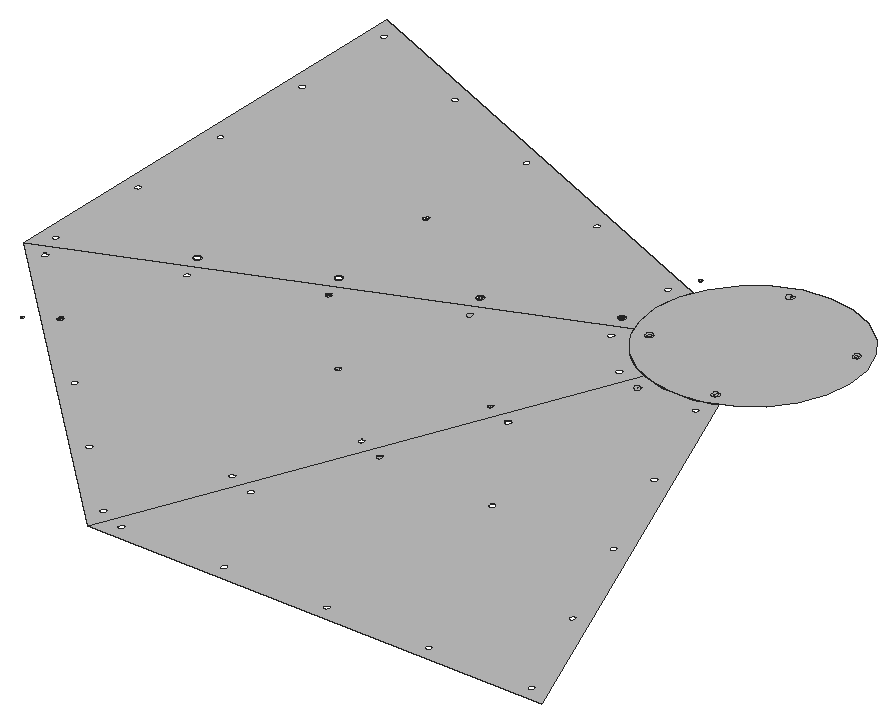
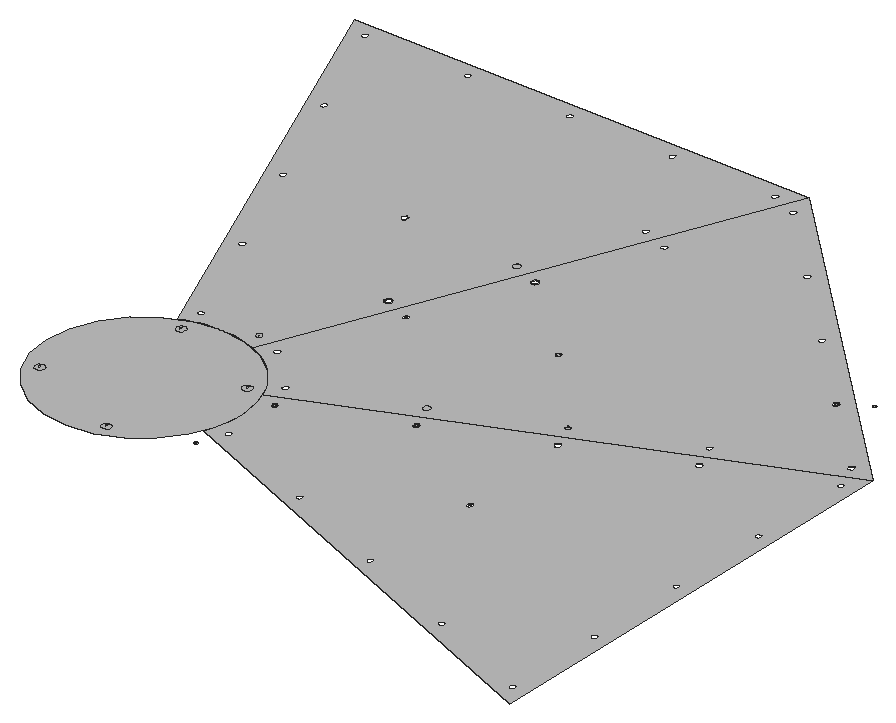
# SketchUp Ruby script. Lengths in inches.
U = 1.inch
M = Sketchup.active_model
def pt(a) = Geom::Point3d.new(a.map { |v| v * U })
def face(e, loops, mat)
  f = e.add_face(loops[0].map { |a| pt(a) })
  loops[1..].each { |l| e.add_face(l.map { |a| pt(a) }).erase! }
  f.material = f.back_material = mat if mat
  f
end
# faces: each face lists its corners as indices into pts; further lists are holes
def faces(e, pts, list, mat = nil) = list.each { |f| face(e, (f[0].is_a?(Array) ? f : [f]).map { |l| l.map { |i| pts[i] } }, mat) }
# xy, xz, yz: faces in a plane at the given z, y or x. An outline is a flat list of corners, or four numbers for a rectangle; further outlines are holes
def ring(l) = l.size == 4 ? [[l[0], l[1]], [l[2], l[1]], [l[2], l[3]], [l[0], l[3]]] : l.each_slice(2).to_a
def flat(e, list, mat, &to3) = list.each { |f| face(e, (f[0].is_a?(Array) ? f : [f]).map { |l| ring(l).map { |u, v| to3.(u, v) } }, mat) }
def xy(e, z, list, mat = nil) = flat(e, list, mat) { |x, y| [x, y, z] }
def xz(e, y, list, mat = nil) = flat(e, list, mat) { |x, z| [x, y, z] }
def yz(e, x, list, mat = nil) = flat(e, list, mat) { |y, z| [x, y, z] }
def lines(e, pts, list) = list.each { |a, b| e.add_line(pt(pts[a]), pt(pts[b])) }
# prism: a flat outline (further loops are holes) pulled along v
def prism(e, loops, v, mat = nil)
  f = face(e, loops, mat); d = Geom::Vector3d.new(v.map { |x| x * U })
  f.pushpull(f.normal.samedirection?(d) ? d.length : -d.length)
end
def box(e, o, s, mat = nil) = prism(e, [[o, [o[0] + s[0], o[1], o[2]], [o[0] + s[0], o[1] + s[1], o[2]], [o[0], o[1] + s[1], o[2]]]], [0, 0, s[2]], mat)
def at(x, y, z, deg = 0) = Geom::Transformation.translation(pt([x, y, z])) * Geom::Transformation.rotation(ORIGIN, Z_AXIS, deg.degrees)
def axes(o, x, y, z) = Geom::Transformation.new([*x, 0, *y, 0, *z, 0, *pt(o).to_a, 1])
def part(name) = M.definitions.add(name)
# library, detail: a bought-in or finely detailed component or shape, given as its bounding box
def library(name, o, s) = part(name).tap { |d| box(d.entities, o, s) }
def detail(e, o, s) = box(e.add_group.entities, o, s)
def put(e, d, t, mat = nil) = e.add_instance(d, t).tap { |i| i.material = mat if mat }
def group(e, t, mat = nil) = e.add_group.tap { |g| g.transformation = t; g.material = mat if mat }.entities
root = M.entities
M.materials.add("[Metal_Steel_Textured_White]").color = [191, 191, 191]
xy(root,3.625,[[[143.617,148.407,134.847,157.176,147.359,162.359,147.431,162.2,147.513,162.047,147.605,161.899,147.706,161.757,147.817,161.623,147.936,161.495,148.063,161.376,148.198,161.266,148.339,161.165,148.487,161.073,148.641,160.99,148.799,160.919],[147.085,157.734,147.108,157.737,147.129,157.746,147.148,157.76,147.162,157.778,147.171,157.8,147.174,157.823,147.171,157.846,147.162,157.867,147.148,157.886,147.129,157.9,147.108,157.909,147.085,157.912,147.062,157.909,147.041,157.9,147.022,157.886,147.008,157.867,146.999,157.846,146.996,157.823,146.999,157.8,147.008,157.778,147.022,157.76,147.041,157.746,147.062,157.737],[141.36,159.353,141.383,159.356,141.404,159.365,141.422,159.379,141.437,159.397,141.445,159.419,141.448,159.442,141.445,159.465,141.437,159.486,141.422,159.505,141.404,159.519,141.383,159.528,141.36,159.531,141.337,159.528,141.315,159.519,141.297,159.505,141.283,159.486,141.274,159.465,141.271,159.442,141.274,159.419,141.283,159.397,141.297,159.379,141.315,159.365,141.337,159.356],[141.495,151.004,141.518,151.007,141.54,151.016,141.558,151.03,141.572,151.048,141.581,151.07,141.584,151.093,141.581,151.116,141.572,151.137,141.558,151.156,141.54,151.17,141.518,151.179,141.495,151.182,141.472,151.179,141.451,151.17,141.433,151.156,141.418,151.137,141.41,151.116,141.407,151.093,141.41,151.07,141.418,151.048,141.433,151.03,141.451,151.016,141.472,151.007],[135.552,156.947,135.575,156.95,135.596,156.959,135.615,156.973,135.629,156.992,135.638,157.013,135.641,157.036,135.638,157.059,135.629,157.081,135.615,157.099,135.596,157.113,135.575,157.122,135.552,157.125,135.529,157.122,135.508,157.113,135.489,157.099,135.475,157.081,135.466,157.059,135.463,157.036,135.466,157.013,135.475,156.992,135.489,156.973,135.508,156.959,135.529,156.95],[144.263,160.556,144.286,160.559,144.308,160.568,144.326,160.582,144.34,160.6,144.349,160.622,144.352,160.645,144.349,160.668,144.34,160.689,144.326,160.707,144.308,160.722,144.286,160.73,144.263,160.733,144.24,160.73,144.219,160.722,144.2,160.707,144.186,160.689,144.177,160.668,144.174,160.645,144.177,160.622,144.186,160.6,144.2,160.582,144.219,160.568,144.24,160.559],[143.477,149.023,143.5,149.026,143.521,149.035,143.539,149.049,143.554,149.067,143.5625,149.088,143.566,149.112,143.5625,149.135,143.554,149.156,143.539,149.174,143.521,149.188,143.5,149.197,143.477,149.2,143.454,149.197,143.432,149.188,143.414,149.174,143.4,149.156,143.391,149.135,143.388,149.112,143.391,149.088,143.4,149.067,143.414,149.049,143.432,149.035,143.454,149.026],[138.456,158.15,138.479,158.153,138.5,158.162,138.519,158.176,138.533,158.195,138.542,158.216,138.545,158.239,138.542,158.262,138.533,158.283,138.519,158.302,138.5,158.316,138.479,158.325,138.456,158.328,138.433,158.325,138.411,158.316,138.393,158.302,138.379,158.283,138.37,158.262,138.367,158.239,138.37,158.216,138.379,158.195,138.393,158.176,138.411,158.162,138.433,158.153],[145.882,154.83,145.905,154.833,145.927,154.842,145.945,154.856,145.959,154.875,145.968,154.896,145.971,154.919,145.968,154.942,145.959,154.964,145.945,154.982,145.927,154.996,145.905,155.005,145.882,155.008,145.859,155.005,145.838,154.996,145.819,154.982,145.805,154.964,145.796,154.942,145.793,154.919,145.796,154.896,145.805,154.875,145.819,154.856,145.838,154.842,145.859,154.833],[148.288,160.638,148.311,160.641,148.332,160.65,148.351,160.664,148.365,160.682,148.374,160.704,148.377,160.727,148.374,160.75,148.365,160.771,148.351,160.79,148.332,160.804,148.311,160.8125,148.288,160.816,148.265,160.8125,148.243,160.804,148.225,160.79,148.211,160.771,148.202,160.75,148.199,160.727,148.202,160.704,148.211,160.682,148.225,160.664,148.243,160.65,148.265,160.641],[147.167,161.758,147.19,161.761,147.212,161.77,147.23,161.784,147.244,161.803,147.253,161.824,147.256,161.847,147.253,161.87,147.244,161.892,147.23,161.91,147.212,161.924,147.19,161.933,147.167,161.936,147.144,161.933,147.123,161.924,147.104,161.91,147.09,161.892,147.081,161.87,147.078,161.847,147.081,161.824,147.09,161.803,147.104,161.784,147.123,161.77,147.144,161.761],[144.679,151.926,144.702,151.929,144.724,151.938,144.742,151.952,144.756,151.971,144.765,151.992,144.768,152.015,144.765,152.038,144.756,152.06,144.742,152.078,144.724,152.092,144.702,152.101,144.679,152.104,144.656,152.101,144.635,152.092,144.617,152.078,144.602,152.06,144.594,152.038,144.591,152.015,144.594,151.992,144.602,151.971,144.617,151.952,144.635,151.938,144.656,151.929],[139.514,152.985,139.537,152.988,139.559,152.997,139.577,153.011,139.591,153.029,139.6,153.051,139.603,153.074,139.6,153.097,139.591,153.118,139.577,153.137,139.559,153.151,139.537,153.16,139.514,153.163,139.491,153.16,139.47,153.151,139.451,153.137,139.4375,153.118,139.428,153.097,139.425,153.074,139.428,153.051,139.4375,153.029,139.451,153.011,139.47,152.997,139.491,152.988],[137.533,154.966,137.556,154.969,137.578,154.978,137.596,154.992,137.61,155.011,137.619,155.032,137.622,155.055,137.619,155.078,137.61,155.099,137.596,155.118,137.578,155.132,137.556,155.141,137.533,155.144,137.51,155.141,137.489,155.132,137.47,155.118,137.456,155.099,137.447,155.078,137.444,155.055,137.447,155.032,137.456,155.011,137.47,154.992,137.489,154.978,137.51,154.969],[143.513,156.984,143.536,156.987,143.558,156.996,143.576,157.01,143.59,157.029,143.599,157.05,143.602,157.073,143.599,157.096,143.59,157.117,143.576,157.136,143.558,157.15,143.536,157.159,143.513,157.162,143.49,157.159,143.469,157.15,143.451,157.136,143.436,157.117,143.428,157.096,143.425,157.073,143.428,157.05,143.436,157.029,143.451,157.01,143.469,156.996,143.49,156.987]],[[143.617,148.407,148.799,160.919,148.962,160.857,149.129,160.807,149.299,160.767,149.471,160.739,149.644,160.722,149.818,160.716,149.992,160.722,150.165,160.739,150.337,160.767,150.507,160.807,150.673,160.857,150.836,160.919,156.019,148.407],[154.219,151.621,154.242,151.624,154.263,151.633,154.282,151.647,154.296,151.665,154.305,151.687,154.308,151.71,154.305,151.733,154.296,151.754,154.282,151.773,154.263,151.787,154.242,151.796,154.219,151.799,154.196,151.796,154.174,151.787,154.156,151.773,154.142,151.754,154.133,151.733,154.13,151.71,154.133,151.687,154.142,151.665,154.156,151.647,154.174,151.633,154.196,151.624],[145.417,151.621,145.44,151.624,145.462,151.633,145.48,151.647,145.494,151.665,145.503,151.687,145.506,151.71,145.503,151.733,145.494,151.754,145.48,151.773,145.462,151.787,145.44,151.796,145.417,151.799,145.394,151.796,145.373,151.787,145.354,151.773,145.34,151.754,145.331,151.733,145.328,151.71,145.331,151.687,145.34,151.665,145.354,151.647,145.373,151.633,145.394,151.624],[149.025,160.332,149.048,160.335,149.07,160.344,149.088,160.358,149.102,160.377,149.111,160.398,149.114,160.421,149.111,160.444,149.102,160.466,149.088,160.484,149.07,160.498,149.048,160.507,149.025,160.51,149.002,160.507,148.981,160.498,148.963,160.484,148.948,160.466,148.94,160.444,148.937,160.421,148.94,160.398,148.948,160.377,148.963,160.358,148.981,160.344,149.002,160.335],[155.421,148.717,155.444,148.72,155.466,148.729,155.484,148.743,155.498,148.762,155.507,148.783,155.51,148.806,155.507,148.829,155.498,148.85,155.484,148.869,155.466,148.883,155.444,148.892,155.421,148.895,155.398,148.892,155.377,148.883,155.359,148.869,155.345,148.85,155.336,148.829,155.333,148.806,155.336,148.783,155.345,148.762,155.359,148.743,155.377,148.729,155.398,148.72],[147.823,157.428,147.846,157.431,147.867,157.44,147.886,157.454,147.9,157.473,147.909,157.494,147.912,157.517,147.909,157.54,147.9,157.562,147.886,157.58,147.867,157.594,147.846,157.603,147.823,157.606,147.8,157.603,147.778,157.594,147.76,157.58,147.746,157.562,147.737,157.54,147.734,157.517,147.737,157.494,147.746,157.473,147.76,157.454,147.778,157.44,147.8,157.431],[144.214,148.717,144.237,148.72,144.259,148.729,144.277,148.743,144.291,148.762,144.3,148.783,144.303,148.806,144.3,148.829,144.291,148.85,144.277,148.869,144.259,148.883,144.237,148.892,144.214,148.895,144.191,148.892,144.17,148.883,144.151,148.869,144.137,148.85,144.128,148.829,144.125,148.806,144.128,148.783,144.137,148.762,144.151,148.743,144.17,148.729,144.191,148.72],[150.61,160.332,150.633,160.335,150.655,160.344,150.673,160.358,150.6875,160.377,150.696,160.398,150.699,160.421,150.696,160.444,150.6875,160.466,150.673,160.484,150.655,160.498,150.633,160.507,150.61,160.51,150.587,160.507,150.566,160.498,150.547,160.484,150.533,160.466,150.524,160.444,150.521,160.421,150.524,160.398,150.533,160.377,150.547,160.358,150.566,160.344,150.587,160.335],[149.818,154.373,149.841,154.376,149.862,154.385,149.881,154.399,149.895,154.417,149.904,154.439,149.907,154.462,149.904,154.485,149.895,154.506,149.881,154.524,149.862,154.539,149.841,154.547,149.818,154.55,149.795,154.547,149.773,154.539,149.755,154.524,149.741,154.506,149.732,154.485,149.729,154.462,149.732,154.439,149.741,154.417,149.755,154.399,149.773,154.385,149.795,154.376],[153.016,154.525,153.039,154.528,153.06,154.537,153.079,154.551,153.093,154.569,153.102,154.591,153.105,154.614,153.102,154.637,153.093,154.658,153.079,154.676,153.06,154.691,153.039,154.699,153.016,154.702,152.993,154.699,152.971,154.691,152.953,154.676,152.939,154.658,152.93,154.637,152.927,154.614,152.93,154.591,152.939,154.569,152.953,154.551,152.971,154.537,152.993,154.528],[147.016,148.717,147.039,148.72,147.061,148.729,147.079,148.743,147.093,148.762,147.102,148.783,147.105,148.806,147.102,148.829,147.093,148.85,147.079,148.869,147.061,148.883,147.039,148.892,147.016,148.895,146.993,148.892,146.972,148.883,146.953,148.869,146.939,148.85,146.93,148.829,146.927,148.806,146.93,148.783,146.939,148.762,146.953,148.743,146.972,148.729,146.993,148.72],[149.818,148.717,149.841,148.72,149.862,148.729,149.881,148.743,149.895,148.762,149.904,148.783,149.907,148.806,149.904,148.829,149.895,148.85,149.881,148.869,149.862,148.883,149.841,148.892,149.818,148.895,149.795,148.892,149.773,148.883,149.755,148.869,149.741,148.85,149.732,148.829,149.729,148.806,149.732,148.783,149.741,148.762,149.755,148.743,149.773,148.729,149.795,148.72],[152.62,148.717,152.643,148.72,152.664,148.729,152.683,148.743,152.697,148.762,152.706,148.783,152.709,148.806,152.706,148.829,152.697,148.85,152.683,148.869,152.664,148.883,152.643,148.892,152.62,148.895,152.597,148.892,152.575,148.883,152.557,148.869,152.543,148.85,152.534,148.829,152.531,148.806,152.534,148.783,152.543,148.762,152.557,148.743,152.575,148.729,152.597,148.72],[146.62,154.525,146.643,154.528,146.664,154.537,146.683,154.551,146.697,154.569,146.706,154.591,146.709,154.614,146.706,154.637,146.697,154.658,146.683,154.676,146.664,154.691,146.643,154.699,146.62,154.702,146.597,154.699,146.575,154.691,146.557,154.676,146.543,154.658,146.534,154.637,146.531,154.614,146.534,154.591,146.543,154.569,146.557,154.551,146.575,154.537,146.597,154.528],[151.813,157.428,151.836,157.431,151.858,157.44,151.876,157.454,151.89,157.473,151.899,157.494,151.902,157.517,151.899,157.54,151.89,157.562,151.876,157.58,151.858,157.594,151.836,157.603,151.813,157.606,151.79,157.603,151.769,157.594,151.75,157.58,151.736,157.562,151.727,157.54,151.724,157.517,151.727,157.494,151.736,157.473,151.75,157.454,151.769,157.44,151.79,157.431]],[149.818,154.373,149.795,154.376,149.773,154.385,149.755,154.399,149.741,154.417,149.732,154.439,149.729,154.462,149.732,154.485,149.741,154.506,149.755,154.524,149.773,154.539,149.795,154.547,149.818,154.55,149.818,154.549,149.795,154.546,149.774,154.538,149.756,154.524,149.742,154.506,149.733,154.484,149.73,154.462,149.733,154.439,149.742,154.418,149.756,154.399,149.774,154.385,149.795,154.377,149.818,154.374],[[146.62,154.525,146.597,154.528,146.575,154.537,146.557,154.551,146.543,154.569,146.534,154.591,146.531,154.614,146.534,154.637,146.543,154.658,146.557,154.676,146.575,154.691,146.597,154.699,146.62,154.702,146.643,154.699,146.664,154.691,146.683,154.676,146.697,154.658,146.706,154.637,146.709,154.614,146.706,154.591,146.697,154.569,146.683,154.551,146.664,154.537,146.643,154.528],[146.62,154.526,146.643,154.529,146.664,154.537,146.682,154.551,146.696,154.57,146.705,154.591,146.708,154.614,146.705,154.636,146.696,154.657,146.682,154.676,146.664,154.69,146.643,154.698,146.62,154.701,146.597,154.698,146.576,154.69,146.558,154.676,146.544,154.657,146.535,154.636,146.532,154.614,146.535,154.591,146.544,154.57,146.558,154.551,146.576,154.537,146.597,154.529]],[[146.62,154.526,146.597,154.529,146.576,154.537,146.558,154.551,146.544,154.57,146.535,154.591,146.532,154.614,146.535,154.636,146.544,154.657,146.558,154.676,146.576,154.69,146.597,154.698,146.62,154.701,146.643,154.698,146.664,154.69,146.682,154.676,146.696,154.657,146.705,154.636,146.708,154.614,146.705,154.591,146.696,154.57,146.682,154.551,146.664,154.537,146.643,154.529],[146.62,154.577,146.629,154.578,146.638,154.582,146.646,154.588,146.652,154.595,146.655,154.604,146.656,154.614,146.655,154.623,146.652,154.632,146.646,154.639,146.638,154.645,146.629,154.649,146.62,154.65,146.61,154.649,146.602,154.645,146.594,154.639,146.588,154.632,146.585,154.623,146.583,154.614,146.585,154.604,146.588,154.595,146.594,154.588,146.602,154.582,146.61,154.578]],
  [[136.852,154.571,136.842,154.572,136.833,154.576,136.826,154.581,136.82,154.589,136.816,154.598,136.815,154.607,136.816,154.617,136.82,154.626,136.826,154.633,136.833,154.639,136.842,154.643,136.852,154.644,136.861,154.643,136.87,154.639,136.878,154.633,136.883,154.626,136.887,154.617,136.888,154.607,136.887,154.598,136.883,154.589,136.878,154.581,136.87,154.576,136.861,154.572],[136.852,154.587,136.857,154.588,136.862,154.59,136.866,154.593,136.869,154.597,136.871,154.602,136.872,154.607,136.871,154.613,136.869,154.617,136.866,154.621,136.862,154.625,136.857,154.627,136.846,154.627,136.842,154.625,136.834,154.617,136.832,154.613,136.832,154.602,136.834,154.597,136.838,154.593,136.842,154.59,136.846,154.588]],[136.852,154.587,136.846,154.588,136.842,154.59,136.838,154.593,136.834,154.597,136.832,154.602,136.832,154.613,136.834,154.617,136.842,154.625,136.846,154.627,136.857,154.627,136.862,154.625,136.866,154.621,136.869,154.617,136.871,154.613,136.872,154.607,136.871,154.602,136.869,154.597,136.866,154.593,136.862,154.59,136.857,154.588],[[145.882,154.83,145.859,154.833,145.838,154.842,145.819,154.856,145.805,154.875,145.796,154.896,145.793,154.919,145.796,154.942,145.805,154.964,145.819,154.982,145.838,154.996,145.859,155.005,145.882,155.008,145.905,155.005,145.927,154.996,145.945,154.982,145.959,154.964,145.968,154.942,145.971,154.919,145.968,154.896,145.959,154.875,145.945,154.856,145.927,154.842,145.905,154.833],[145.882,154.831,145.905,154.834,145.926,154.843,145.944,154.857,145.958,154.875,145.967,154.896,145.97,154.919,145.967,154.942,145.958,154.963,145.944,154.981,145.926,154.995,145.905,155.004,145.882,155.007,145.859,155.004,145.838,154.995,145.82,154.981,145.806,154.963,145.797,154.942,145.794,154.919,145.797,154.896,145.806,154.875,145.82,154.857,145.838,154.843,145.859,154.834]],[[137.533,154.966,137.51,154.969,137.489,154.978,137.47,154.992,137.456,155.011,137.447,155.032,137.444,155.055,137.447,155.078,137.456,155.099,137.47,155.118,137.489,155.132,137.51,155.141,137.533,155.144,137.556,155.141,137.578,155.132,137.596,155.118,137.61,155.099,137.619,155.078,137.622,155.055,137.619,155.032,137.61,155.011,137.596,154.992,137.578,154.978,137.556,154.969],[137.533,154.967,137.556,154.97,137.577,154.979,137.595,154.993,137.609,155.011,137.618,155.032,137.621,155.055,137.618,155.078,137.609,155.099,137.595,155.117,137.577,155.131,137.556,155.14,137.533,155.143,137.51,155.14,137.489,155.131,137.471,155.117,137.457,155.099,137.448,155.078,137.445,155.055,137.448,155.032,137.457,155.011,137.471,154.993,137.489,154.979,137.51,154.97]],[[137.533,155.018,137.524,155.02,137.515,155.023,137.507,155.029,137.501,155.037,137.498,155.046,137.497,155.055,137.498,155.064,137.501,155.073,137.507,155.081,137.515,155.087,137.524,155.09,137.533,155.092,137.543,155.09,137.551,155.087,137.559,155.081,137.565,155.073,137.568,155.064,137.57,155.055,137.568,155.046,137.565,155.037,137.559,155.029,137.551,155.023,137.543,155.02],[137.533,155.035,137.538,155.036,137.543,155.038,137.547,155.041,137.55,155.045,137.552,155.05,137.553,155.055,137.552,155.06,137.55,155.065,137.547,155.069,137.543,155.072,137.538,155.074,137.533,155.075,137.528,155.074,137.523,155.072,137.519,155.069,137.516,155.065,137.514,155.06,137.513,155.055,137.514,155.05,137.516,155.045,137.519,155.041,137.523,155.038,137.528,155.036]],
  [137.533,155.035,137.528,155.036,137.523,155.038,137.519,155.041,137.516,155.045,137.514,155.05,137.513,155.055,137.514,155.06,137.516,155.065,137.519,155.069,137.523,155.072,137.528,155.074,137.533,155.075,137.538,155.074,137.543,155.072,137.547,155.069,137.55,155.065,137.552,155.06,137.553,155.055,137.552,155.05,137.55,155.045,137.547,155.041,137.543,155.038,137.538,155.036],[[135.552,156.947,135.529,156.95,135.508,156.959,135.489,156.973,135.475,156.992,135.466,157.013,135.463,157.036,135.466,157.059,135.475,157.081,135.489,157.099,135.508,157.113,135.529,157.122,135.552,157.125,135.575,157.122,135.596,157.113,135.615,157.099,135.629,157.081,135.638,157.059,135.641,157.036,135.638,157.013,135.629,156.992,135.615,156.973,135.596,156.959,135.575,156.95],[135.552,156.948,135.575,156.951,135.596,156.96,135.614,156.974,135.628,156.992,135.637,157.013,135.64,157.036,135.637,157.059,135.628,157.08,135.614,157.098,135.596,157.112,135.575,157.121,135.552,157.124,135.529,157.121,135.508,157.112,135.49,157.098,135.476,157.08,135.467,157.059,135.464,157.036,135.467,157.013,135.476,156.992,135.49,156.974,135.508,156.96,135.529,156.951]],[[143.513,157.036,143.504,157.038,143.495,157.041,143.488,157.047,143.482,157.055,143.478,157.063,143.477,157.073,143.478,157.082,143.482,157.091,143.488,157.099,143.495,157.105,143.504,157.108,143.513,157.11,143.523,157.108,143.532,157.105,143.539,157.099,143.545,157.091,143.549,157.082,143.55,157.073,143.549,157.063,143.545,157.055,143.539,157.047,143.532,157.041,143.523,157.038],[143.513,157.053,143.519,157.054,143.523,157.056,143.528,157.059,143.531,157.063,143.533,157.068,143.533,157.078,143.531,157.083,143.528,157.087,143.523,157.09,143.519,157.092,143.513,157.093,143.508,157.092,143.503,157.09,143.499,157.087,143.496,157.083,143.494,157.078,143.493,157.073,143.494,157.068,143.496,157.063,143.499,157.059,143.503,157.056,143.508,157.054]],[[134.847,157.176,134.847,169.578,147.359,164.396,147.298,164.233,147.247,164.066,147.208,163.897,147.179,163.725,147.162,163.551,147.156,163.377,147.162,163.203,147.179,163.03,147.208,162.858,147.247,162.689,147.298,162.522,147.359,162.359],[143.958,161.293,143.981,161.296,144.002,161.305,144.021,161.319,144.035,161.338,144.044,161.359,144.047,161.382,144.044,161.405,144.035,161.427,144.021,161.445,144.002,161.459,143.981,161.468,143.958,161.471,143.935,161.468,143.913,161.459,143.895,161.445,143.881,161.427,143.872,161.405,143.869,161.382,143.872,161.359,143.881,161.338,143.895,161.319,143.913,161.305,143.935,161.296],[135.246,168.892,135.269,168.895,135.291,168.904,135.309,168.918,135.323,168.937,135.332,168.958,135.335,168.981,135.332,169.004,135.323,169.025,135.309,169.044,135.291,169.058,135.269,169.067,135.246,169.07,135.223,169.067,135.202,169.058,135.184,169.044,135.169,169.025,135.161,169.004,135.158,168.981,135.161,168.958,135.169,168.937,135.184,168.918,135.202,168.904,135.223,168.895],[135.246,160.487,135.269,160.49,135.291,160.499,135.309,160.513,135.323,160.531,135.332,160.553,135.335,160.576,135.332,160.599,135.323,160.62,135.309,160.638,135.291,160.653,135.269,160.661,135.246,160.665,135.223,160.661,135.202,160.653,135.184,160.638,135.169,160.62,135.161,160.599,135.158,160.576,135.161,160.553,135.169,160.531,135.184,160.513,135.202,160.499,135.223,160.49],[135.246,166.09,135.269,166.093,135.291,166.102,135.309,166.116,135.323,166.135,135.332,166.156,135.335,166.179,135.332,166.202,135.323,166.224,135.309,166.242,135.291,166.256,135.269,166.265,135.246,166.268,135.223,166.265,135.202,166.256,135.184,166.242,135.169,166.224,135.161,166.202,135.158,166.179,135.161,166.156,135.169,166.135,135.184,166.116,135.202,166.102,135.223,166.093],[141.054,166.487,141.077,166.49,141.098,166.498,141.117,166.513,141.131,166.531,141.14,166.552,141.143,166.575,141.14,166.598,141.131,166.62,141.117,166.638,141.098,166.652,141.077,166.661,141.054,166.664,141.031,166.661,141.01,166.652,140.991,166.638,140.977,166.62,140.968,166.598,140.965,166.575,140.968,166.552,140.977,166.531,140.991,166.513,141.01,166.498,141.031,166.49],[135.246,157.685,135.269,157.688,135.291,157.697,135.309,157.711,135.323,157.729,135.332,157.751,135.335,157.774,135.332,157.797,135.323,157.818,135.309,157.837,135.291,157.851,135.269,157.86,135.246,157.863,135.223,157.86,135.202,157.851,135.184,157.837,135.169,157.818,135.161,157.797,135.158,157.774,135.161,157.751,135.169,157.729,135.184,157.711,135.202,157.697,135.223,157.688],[135.246,163.289,135.269,163.292,135.291,163.3,135.309,163.315,135.323,163.333,135.332,163.354,135.335,163.377,135.332,163.4,135.323,163.422,135.309,163.44,135.291,163.454,135.269,163.463,135.246,163.466,135.223,163.463,135.202,163.454,135.184,163.44,135.169,163.422,135.161,163.4,135.158,163.377,135.161,163.354,135.169,163.333,135.184,163.315,135.202,163.3,135.223,163.292],[146.862,164.081,146.885,164.084,146.906,164.093,146.924,164.107,146.939,164.125,146.947,164.147,146.95,164.17,146.947,164.193,146.939,164.214,146.924,164.233,146.906,164.247,146.885,164.256,146.862,164.259,146.839,164.256,146.817,164.247,146.799,164.233,146.785,164.214,146.776,164.193,146.773,164.17,146.776,164.147,146.785,164.125,146.799,164.107,146.817,164.093,146.839,164.084],[146.862,162.496,146.885,162.499,146.906,162.508,146.924,162.522,146.939,162.541,146.947,162.562,146.95,162.585,146.947,162.608,146.939,162.629,146.924,162.648,146.906,162.662,146.885,162.671,146.862,162.674,146.839,162.671,146.817,162.662,146.799,162.648,146.785,162.629,146.776,162.608,146.773,162.585,146.776,162.562,146.785,162.541,146.799,162.522,146.817,162.508,146.839,162.499],[140.902,163.289,140.925,163.292,140.946,163.3,140.965,163.315,140.979,163.333,140.988,163.354,140.991,163.377,140.988,163.4,140.979,163.422,140.965,163.44,140.946,163.454,140.925,163.463,140.902,163.466,140.879,163.463,140.858,163.454,140.839,163.44,140.825,163.422,140.816,163.4,140.813,163.377,140.816,163.354,140.825,163.333,140.839,163.315,140.858,163.3,140.879,163.292],[138.15,158.888,138.173,158.891,138.195,158.9,138.213,158.914,138.227,158.932,138.236,158.954,138.239,158.977,138.236,159,138.227,159.021,138.213,159.039,138.195,159.054,138.173,159.0625,138.15,159.066,138.127,159.0625,138.106,159.054,138.087,159.039,138.073,159.021,138.064,159,138.061,158.977,138.064,158.954,138.073,158.932,138.087,158.914,138.106,158.9,138.127,158.891],[138.15,167.689,138.173,167.692,138.195,167.701,138.213,167.715,138.227,167.734,138.236,167.755,138.239,167.778,138.236,167.801,138.227,167.823,138.213,167.841,138.195,167.855,138.173,167.864,138.15,167.867,138.127,167.864,138.106,167.855,138.087,167.841,138.073,167.823,138.064,167.801,138.061,167.778,138.064,167.755,138.073,167.734,138.087,167.715,138.106,167.701,138.127,167.692],[141.054,160.091,141.077,160.094,141.098,160.102,141.117,160.117,141.131,160.135,141.14,160.156,141.143,160.179,141.14,160.202,141.131,160.224,141.117,160.242,141.098,160.256,141.077,160.265,141.054,160.268,141.031,160.265,141.01,160.256,140.991,160.242,140.977,160.224,140.968,160.202,140.965,160.179,140.968,160.156,140.977,160.135,140.991,160.117,141.01,160.102,141.031,160.094],[143.958,165.284,143.981,165.287,144.002,165.296,144.021,165.31,144.035,165.328,144.044,165.35,144.047,165.373,144.044,165.396,144.035,165.417,144.021,165.435,144.002,165.45,143.981,165.459,143.958,165.462,143.935,165.459,143.913,165.45,143.895,165.435,143.881,165.417,143.872,165.396,143.869,165.373,143.872,165.35,143.881,165.328,143.895,165.31,143.913,165.296,143.935,165.287]],[[147.823,157.428,147.8,157.431,147.778,157.44,147.76,157.454,147.746,157.473,147.737,157.494,147.734,157.517,147.737,157.54,147.746,157.562,147.76,157.58,147.778,157.594,147.8,157.603,147.823,157.606,147.846,157.603,147.867,157.594,147.886,157.58,147.9,157.562,147.909,157.54,147.912,157.517,147.909,157.494,147.9,157.473,147.886,157.454,147.867,157.44,147.846,157.431],[147.823,157.429,147.845,157.432,147.867,157.441,147.885,157.455,147.899,157.473,147.908,157.495,147.911,157.517,147.908,157.54,147.899,157.561,147.885,157.579,147.867,157.593,147.845,157.602,147.823,157.605,147.8,157.602,147.779,157.593,147.76,157.579,147.747,157.561,147.738,157.54,147.735,157.517,147.738,157.495,147.747,157.473,147.76,157.455,147.779,157.441,147.8,157.432]],
  [[147.085,157.786,147.076,157.788,147.067,157.791,147.059,157.797,147.053,157.805,147.05,157.813,147.048,157.823,147.05,157.832,147.053,157.841,147.059,157.849,147.067,157.855,147.076,157.858,147.085,157.859,147.094,157.858,147.103,157.855,147.111,157.849,147.117,157.841,147.12,157.832,147.122,157.823,147.12,157.813,147.117,157.805,147.111,157.797,147.103,157.791,147.094,157.788],[147.085,157.803,147.09,157.804,147.095,157.806,147.099,157.809,147.102,157.813,147.104,157.818,147.105,157.823,147.104,157.828,147.102,157.833,147.099,157.837,147.095,157.84,147.09,157.842,147.085,157.843,147.08,157.842,147.075,157.84,147.071,157.837,147.068,157.833,147.066,157.828,147.065,157.823,147.066,157.818,147.068,157.813,147.071,157.809,147.075,157.806,147.08,157.804]],[147.085,157.803,147.08,157.804,147.075,157.806,147.071,157.809,147.068,157.813,147.066,157.818,147.065,157.823,147.066,157.828,147.068,157.833,147.071,157.837,147.075,157.84,147.08,157.842,147.085,157.843,147.09,157.842,147.095,157.84,147.099,157.837,147.102,157.833,147.104,157.828,147.105,157.823,147.104,157.818,147.102,157.813,147.099,157.809,147.095,157.806,147.09,157.804],[[138.15,158.888,138.127,158.891,138.106,158.9,138.087,158.914,138.073,158.932,138.064,158.954,138.061,158.977,138.064,159,138.073,159.021,138.087,159.039,138.106,159.054,138.127,159.0625,138.15,159.066,138.173,159.0625,138.195,159.054,138.213,159.039,138.227,159.021,138.236,159,138.239,158.977,138.236,158.954,138.227,158.932,138.213,158.914,138.195,158.9,138.173,158.891],[138.15,158.889,138.173,158.892,138.194,158.9,138.212,158.914,138.226,158.933,138.235,158.954,138.238,158.977,138.235,158.999,138.226,159.021,138.212,159.039,138.194,159.053,138.173,159.062,138.15,159.065,138.127,159.062,138.106,159.053,138.088,159.039,138.074,159.021,138.065,158.999,138.062,158.977,138.065,158.954,138.074,158.933,138.088,158.914,138.106,158.9,138.127,158.892]],[[141.36,159.354,141.337,159.357,141.316,159.366,141.297,159.38,141.283,159.398,141.275,159.419,141.272,159.442,141.275,159.465,141.283,159.486,141.297,159.504,141.316,159.518,141.337,159.527,141.36,159.53,141.382,159.527,141.404,159.518,141.422,159.504,141.436,159.486,141.444,159.465,141.447,159.442,141.444,159.419,141.436,159.398,141.422,159.38,141.404,159.366,141.382,159.357],[141.36,159.405,141.369,159.406,141.378,159.41,141.385,159.416,141.391,159.423,141.395,159.432,141.396,159.442,141.395,159.451,141.391,159.46,141.385,159.468,141.378,159.473,141.369,159.477,141.36,159.478,141.35,159.477,141.341,159.473,141.334,159.468,141.328,159.46,141.324,159.451,141.323,159.442,141.324,159.432,141.328,159.423,141.334,159.416,141.341,159.41,141.35,159.406]],[[141.36,159.405,141.35,159.406,141.341,159.41,141.334,159.416,141.328,159.423,141.324,159.432,141.323,159.442,141.324,159.451,141.328,159.46,141.334,159.468,141.341,159.473,141.35,159.477,141.36,159.478,141.369,159.477,141.378,159.473,141.385,159.468,141.391,159.46,141.395,159.451,141.396,159.442,141.395,159.432,141.391,159.423,141.385,159.416,141.378,159.41,141.369,159.406],[141.354,159.422,141.365,159.422,141.37,159.424,141.374,159.428,141.377,159.432,141.379,159.437,141.38,159.442,141.379,159.447,141.377,159.452,141.374,159.456,141.37,159.459,141.365,159.461,141.36,159.462,141.354,159.461,141.35,159.459,141.345,159.456,141.342,159.452,141.34,159.447,141.34,159.437,141.342,159.432,141.345,159.428,141.35,159.424]],
  [[141.054,160.091,141.031,160.094,141.01,160.102,140.991,160.117,140.977,160.135,140.968,160.156,140.965,160.179,140.968,160.202,140.977,160.224,140.991,160.242,141.01,160.256,141.031,160.265,141.054,160.268,141.077,160.265,141.098,160.256,141.117,160.242,141.131,160.224,141.14,160.202,141.143,160.179,141.14,160.156,141.131,160.135,141.117,160.117,141.098,160.102,141.077,160.094],[141.054,160.091,141.077,160.094,141.098,160.103,141.116,160.117,141.13,160.135,141.139,160.157,141.142,160.179,141.139,160.202,141.13,160.223,141.116,160.242,141.098,160.256,141.077,160.264,141.054,160.267,141.031,160.264,141.01,160.256,140.992,160.242,140.978,160.223,140.969,160.202,140.966,160.179,140.969,160.157,140.978,160.135,140.992,160.117,141.01,160.103,141.031,160.094]],[[149.025,160.333,149.003,160.336,148.981,160.345,148.963,160.359,148.949,160.377,148.941,160.398,148.9375,160.421,148.941,160.444,148.949,160.465,148.963,160.483,148.981,160.497,149.003,160.506,149.025,160.509,149.048,160.506,149.069,160.497,149.088,160.483,149.102,160.465,149.11,160.444,149.113,160.421,149.11,160.398,149.102,160.377,149.088,160.359,149.069,160.345,149.048,160.336],[149.025,160.385,149.035,160.386,149.044,160.389,149.051,160.395,149.057,160.403,149.061,160.412,149.062,160.421,149.061,160.431,149.057,160.439,149.051,160.447,149.044,160.453,149.035,160.456,149.025,160.458,149.016,160.456,149.007,160.453,149,160.447,148.994,160.439,148.99,160.431,148.989,160.421,148.99,160.412,148.994,160.403,149,160.395,149.007,160.389,149.016,160.386]],[[144.263,160.557,144.241,160.56,144.219,160.568,144.201,160.582,144.187,160.601,144.178,160.622,144.175,160.645,144.178,160.667,144.187,160.689,144.201,160.707,144.219,160.721,144.241,160.729,144.263,160.732,144.286,160.729,144.307,160.721,144.326,160.707,144.339,160.689,144.348,160.667,144.351,160.645,144.348,160.622,144.339,160.601,144.326,160.582,144.307,160.568,144.286,160.56],[144.263,160.608,144.273,160.609,144.282,160.613,144.289,160.619,144.295,160.626,144.299,160.635,144.3,160.645,144.299,160.654,144.295,160.663,144.289,160.67,144.282,160.676,144.273,160.68,144.263,160.681,144.254,160.68,144.245,160.676,144.237,160.67,144.232,160.663,144.228,160.654,144.227,160.645,144.228,160.635,144.232,160.626,144.237,160.619,144.245,160.613,144.254,160.609]],[[149.818,160.729,149.133,160.82,148.494,161.084,147.945,161.505,147.525,162.053,147.26,162.692,147.17,163.377,147.26,164.063,147.525,164.701,147.945,165.25,148.494,165.671,149.133,165.935,149.818,166.026,150.503,165.935,151.142,165.671,151.69,165.25,152.111,164.701,152.376,164.063,152.466,163.377,152.376,162.692,152.111,162.053,151.69,161.505,151.142,161.084,150.503,160.82],[149.119,165.409,149.15,165.413,149.179,165.425,149.204,165.444,149.223,165.469,149.235,165.498,149.239,165.529,149.235,165.56,149.223,165.589,149.204,165.614,149.179,165.633,149.15,165.645,149.119,165.649,149.088,165.645,149.059,165.633,149.034,165.614,149.015,165.589,149.003,165.56,148.999,165.529,149.003,165.498,149.015,165.469,149.034,165.444,149.059,165.425,149.088,165.413],[150.517,161.106,150.548,161.11,150.577,161.122,150.602,161.141,150.621,161.166,150.633,161.195,150.637,161.226,150.633,161.257,150.621,161.286,150.602,161.311,150.577,161.33,150.548,161.342,150.517,161.346,150.486,161.342,150.457,161.33,150.432,161.311,150.413,161.286,150.401,161.257,150.397,161.226,150.401,161.195,150.413,161.166,150.432,161.141,150.457,161.122,150.486,161.11],[151.834,164.285,151.865,164.289,151.893,164.301,151.918,164.32,151.937,164.345,151.949,164.373,151.953,164.404,151.949,164.435,151.937,164.464,151.918,164.489,151.893,164.508,151.865,164.52,151.834,164.524,151.803,164.52,151.774,164.508,151.749,164.489,151.73,164.464,151.718,164.435,151.714,164.404,151.718,164.373,151.73,164.345,151.749,164.32,151.774,164.301,151.803,164.289],[147.802,162.231,147.833,162.235,147.862,162.247,147.887,162.266,147.906,162.291,147.918,162.319,147.922,162.35,147.918,162.381,147.906,162.41,147.887,162.435,147.862,162.454,147.833,162.466,147.802,162.47,147.771,162.466,147.742,162.454,147.718,162.435,147.699,162.41,147.687,162.381,147.682,162.35,147.687,162.319,147.699,162.291,147.718,162.266,147.742,162.247,147.771,162.235]],[[150.517,161.106,150.486,161.11,150.457,161.122,150.432,161.141,150.413,161.166,150.401,161.195,150.397,161.226,150.401,161.257,150.413,161.286,150.432,161.311,150.457,161.33,150.486,161.342,150.517,161.346,150.548,161.342,150.577,161.33,150.602,161.311,150.621,161.286,150.633,161.257,150.637,161.226,150.633,161.195,150.621,161.166,150.602,161.141,150.577,161.122,150.548,161.11],[150.514,161.18,150.52,161.182,150.525,161.185,150.535,161.19,150.545,161.196,150.55,161.198,150.556,161.201,150.556,161.212,150.557,161.218,150.557,161.235,150.558,161.241,150.558,161.247,150.548,161.253,150.544,161.256,150.534,161.262,150.529,161.266,150.524,161.269,150.52,161.272,150.514,161.269,150.509,161.267,150.504,161.264,150.499,161.262,150.489,161.256,150.483,161.254,150.478,161.251,150.478,161.24,150.477,161.234,150.477,161.222,150.476,161.217,150.476,161.205,150.481,161.202,150.485,161.199,150.49,161.196,150.495,161.192,150.51,161.183]],
  [150.514,161.18,150.51,161.183,150.495,161.192,150.49,161.196,150.485,161.199,150.481,161.202,150.476,161.205,150.476,161.217,150.477,161.222,150.477,161.234,150.478,161.24,150.478,161.251,150.483,161.254,150.489,161.256,150.499,161.262,150.504,161.264,150.509,161.267,150.514,161.269,150.52,161.272,150.524,161.269,150.529,161.266,150.534,161.262,150.544,161.256,150.548,161.253,150.558,161.247,150.558,161.241,150.557,161.235,150.557,161.218,150.556,161.212,150.556,161.201,150.55,161.198,150.545,161.196,150.535,161.19,150.525,161.185,150.52,161.182],[[143.958,161.293,143.935,161.296,143.913,161.305,143.895,161.319,143.881,161.338,143.872,161.359,143.869,161.382,143.872,161.405,143.881,161.427,143.895,161.445,143.913,161.459,143.935,161.468,143.958,161.471,143.981,161.468,144.002,161.459,144.021,161.445,144.035,161.427,144.044,161.405,144.047,161.382,144.044,161.359,144.035,161.338,144.021,161.319,144.002,161.305,143.981,161.296],[143.958,161.294,143.981,161.297,144.002,161.306,144.02,161.32,144.034,161.338,144.043,161.359,144.046,161.382,144.043,161.405,144.034,161.426,144.02,161.444,144.002,161.458,143.981,161.467,143.958,161.47,143.935,161.467,143.914,161.458,143.896,161.444,143.882,161.426,143.873,161.405,143.87,161.382,143.873,161.359,143.882,161.338,143.896,161.32,143.914,161.306,143.935,161.297]],[[143.958,161.346,143.948,161.347,143.939,161.351,143.932,161.356,143.926,161.364,143.922,161.373,143.921,161.382,143.922,161.392,143.926,161.4,143.932,161.408,143.939,161.414,143.948,161.418,143.958,161.419,143.967,161.418,143.976,161.414,143.984,161.408,143.989,161.4,143.993,161.392,143.994,161.382,143.993,161.373,143.989,161.364,143.984,161.356,143.976,161.351,143.967,161.347],[143.958,161.362,143.963,161.363,143.968,161.365,143.972,161.368,143.975,161.372,143.977,161.377,143.978,161.382,143.977,161.387,143.975,161.392,143.972,161.396,143.968,161.399,143.963,161.401,143.958,161.402,143.953,161.401,143.948,161.399,143.944,161.396,143.941,161.392,143.939,161.387,143.938,161.382,143.939,161.377,143.941,161.372,143.944,161.368,143.948,161.365,143.953,161.363]],[143.958,161.362,143.953,161.363,143.948,161.365,143.944,161.368,143.941,161.372,143.939,161.377,143.938,161.382,143.939,161.387,143.941,161.392,143.944,161.396,143.948,161.399,143.953,161.401,143.958,161.402,143.963,161.401,143.968,161.399,143.972,161.396,143.975,161.392,143.977,161.387,143.978,161.382,143.977,161.377,143.975,161.372,143.972,161.368,143.968,161.365,143.963,161.363],[[147.802,162.231,147.771,162.235,147.742,162.247,147.718,162.266,147.699,162.291,147.687,162.319,147.682,162.35,147.687,162.381,147.699,162.41,147.718,162.435,147.742,162.454,147.771,162.466,147.802,162.47,147.833,162.466,147.862,162.454,147.887,162.435,147.906,162.41,147.918,162.381,147.922,162.35,147.918,162.319,147.906,162.291,147.887,162.266,147.862,162.247,147.833,162.235],[147.8,162.304,147.81,162.31,147.815,162.312,147.82,162.315,147.825,162.317,147.831,162.32,147.836,162.323,147.841,162.325,147.841,162.337,147.842,162.342,147.842,162.354,147.843,162.36,147.843,162.371,147.839,162.374,147.834,162.377,147.829,162.381,147.814,162.39,147.81,162.393,147.805,162.396,147.8,162.394,147.795,162.391,147.789,162.389,147.779,162.383,147.774,162.381,147.769,162.378,147.764,162.376,147.763,162.37,147.763,162.358,147.762,162.353,147.762,162.341,147.761,162.335,147.761,162.33,147.766,162.326,147.776,162.32,147.78,162.317,147.79,162.311,147.795,162.307]],
  [147.8,162.304,147.795,162.307,147.79,162.311,147.78,162.317,147.776,162.32,147.766,162.326,147.761,162.33,147.761,162.335,147.762,162.341,147.762,162.353,147.763,162.358,147.763,162.37,147.764,162.376,147.769,162.378,147.774,162.381,147.779,162.383,147.789,162.389,147.795,162.391,147.8,162.394,147.805,162.396,147.81,162.393,147.814,162.39,147.829,162.381,147.834,162.377,147.839,162.374,147.843,162.371,147.843,162.36,147.842,162.354,147.842,162.342,147.841,162.337,147.841,162.325,147.836,162.323,147.831,162.32,147.825,162.317,147.82,162.315,147.815,162.312,147.81,162.31],[[146.862,162.496,146.839,162.499,146.817,162.508,146.799,162.522,146.785,162.541,146.776,162.562,146.773,162.585,146.776,162.608,146.785,162.629,146.799,162.648,146.817,162.662,146.839,162.671,146.862,162.674,146.885,162.671,146.906,162.662,146.924,162.648,146.939,162.629,146.947,162.608,146.95,162.585,146.947,162.562,146.939,162.541,146.924,162.522,146.906,162.508,146.885,162.499],[146.862,162.497,146.884,162.5,146.906,162.509,146.924,162.523,146.938,162.541,146.947,162.562,146.95,162.585,146.947,162.608,146.938,162.629,146.924,162.647,146.906,162.661,146.884,162.67,146.862,162.673,146.839,162.67,146.818,162.661,146.799,162.647,146.785,162.629,146.777,162.608,146.774,162.585,146.777,162.562,146.785,162.541,146.799,162.523,146.818,162.509,146.839,162.5]],[[146.862,162.548,146.852,162.55,146.843,162.553,146.836,162.559,146.83,162.567,146.826,162.576,146.825,162.585,146.826,162.594,146.83,162.603,146.836,162.611,146.843,162.617,146.852,162.62,146.862,162.622,146.871,162.62,146.88,162.617,146.887,162.611,146.893,162.603,146.897,162.594,146.898,162.585,146.897,162.576,146.893,162.567,146.887,162.559,146.88,162.553,146.871,162.55],[146.862,162.565,146.867,162.566,146.872,162.568,146.876,162.571,146.879,162.575,146.881,162.58,146.882,162.585,146.881,162.59,146.879,162.595,146.876,162.599,146.872,162.602,146.867,162.604,146.862,162.605,146.856,162.604,146.852,162.602,146.847,162.599,146.844,162.595,146.842,162.59,146.842,162.58,146.844,162.575,146.847,162.571,146.852,162.568,146.856,162.566]],[146.862,162.565,146.856,162.566,146.852,162.568,146.847,162.571,146.844,162.575,146.842,162.58,146.842,162.59,146.844,162.595,146.847,162.599,146.852,162.602,146.856,162.604,146.862,162.605,146.867,162.604,146.872,162.602,146.876,162.599,146.879,162.595,146.881,162.59,146.882,162.585,146.881,162.58,146.879,162.575,146.876,162.571,146.872,162.568,146.867,162.566],[140.902,163.289,140.879,163.292,140.858,163.3,140.839,163.315,140.825,163.333,140.816,163.354,140.813,163.377,140.814,163.377,140.817,163.355,140.826,163.333,140.84,163.315,140.858,163.301,140.879,163.292,140.902,163.289,140.925,163.292,140.946,163.301,140.964,163.315,140.978,163.333,140.987,163.355,140.99,163.377,140.991,163.377,140.988,163.354,140.979,163.333,140.965,163.315,140.946,163.3,140.925,163.292],
  [140.902,163.357,140.897,163.358,140.892,163.36,140.888,163.363,140.885,163.367,140.883,163.372,140.882,163.377,140.922,163.377,140.921,163.372,140.919,163.367,140.916,163.363,140.912,163.36,140.907,163.358],[[151.834,164.285,151.803,164.289,151.774,164.301,151.749,164.32,151.73,164.345,151.718,164.373,151.714,164.404,151.718,164.435,151.73,164.464,151.749,164.489,151.774,164.508,151.803,164.52,151.834,164.524,151.865,164.52,151.893,164.508,151.918,164.489,151.937,164.464,151.949,164.435,151.953,164.404,151.949,164.373,151.937,164.345,151.918,164.32,151.893,164.301,151.865,164.289],[151.831,164.358,151.841,164.364,151.846,164.366,151.852,164.369,151.857,164.371,151.867,164.377,151.872,164.379,151.872,164.385,151.873,164.391,151.873,164.402,151.874,164.408,151.874,164.42,151.875,164.425,151.87,164.428,151.865,164.432,151.855,164.438,151.851,164.441,151.836,164.45,151.831,164.448,151.826,164.445,151.821,164.443,151.816,164.44,151.81,164.4375,151.805,164.435,151.8,164.432,151.795,164.43,151.795,164.424,151.794,164.418,151.794,164.407,151.793,164.401,151.793,164.389,151.792,164.384,151.797,164.381,151.802,164.377,151.817,164.368,151.821,164.365,151.826,164.362]],[151.831,164.358,151.826,164.362,151.821,164.365,151.817,164.368,151.802,164.377,151.797,164.381,151.792,164.384,151.793,164.389,151.793,164.401,151.794,164.407,151.794,164.418,151.795,164.424,151.795,164.43,151.8,164.432,151.805,164.435,151.81,164.4375,151.816,164.44,151.821,164.443,151.826,164.445,151.831,164.448,151.836,164.45,151.851,164.441,151.855,164.438,151.865,164.432,151.87,164.428,151.875,164.425,151.874,164.42,151.874,164.408,151.873,164.402,151.873,164.391,151.872,164.385,151.872,164.379,151.867,164.377,151.857,164.371,151.852,164.369,151.846,164.366,151.841,164.364],[[147.167,164.871,147.158,164.872,147.149,164.876,147.141,164.882,147.135,164.889,147.132,164.898,147.131,164.908,147.132,164.917,147.135,164.926,147.141,164.933,147.149,164.939,147.158,164.943,147.167,164.944,147.177,164.943,147.185,164.939,147.193,164.933,147.199,164.926,147.202,164.917,147.204,164.908,147.202,164.898,147.199,164.889,147.193,164.882,147.185,164.876,147.177,164.872],[147.162,164.888,147.172,164.888,147.177,164.89,147.181,164.893,147.184,164.898,147.186,164.902,147.187,164.908,147.186,164.913,147.184,164.917,147.181,164.922,147.177,164.925,147.172,164.927,147.162,164.927,147.157,164.925,147.153,164.922,147.15,164.917,147.148,164.913,147.147,164.908,147.148,164.902,147.15,164.898,147.153,164.893,147.157,164.89]],[147.162,164.888,147.157,164.89,147.153,164.893,147.15,164.898,147.148,164.902,147.147,164.908,147.148,164.913,147.15,164.917,147.153,164.922,147.157,164.925,147.162,164.927,147.172,164.927,147.177,164.925,147.181,164.922,147.184,164.917,147.186,164.913,147.187,164.908,147.186,164.902,147.184,164.898,147.181,164.893,147.177,164.89,147.172,164.888],
  [[149.119,165.409,149.088,165.413,149.059,165.425,149.034,165.444,149.015,165.469,149.003,165.498,148.999,165.529,149.003,165.56,149.015,165.589,149.034,165.614,149.059,165.633,149.088,165.645,149.119,165.649,149.15,165.645,149.179,165.633,149.204,165.614,149.223,165.589,149.235,165.56,149.239,165.529,149.235,165.498,149.223,165.469,149.204,165.444,149.179,165.425,149.15,165.413],[149.116,165.483,149.121,165.485,149.127,165.488,149.132,165.491,149.137,165.493,149.147,165.499,149.152,165.501,149.157,165.504,149.158,165.509,149.158,165.521,149.159,165.527,149.159,165.538,149.16,165.544,149.16,165.55,149.15,165.556,149.146,165.559,149.136,165.566,149.121,165.575,149.116,165.572,149.111,165.57,149.106,165.567,149.101,165.565,149.096,165.562,149.09,165.559,149.085,165.557,149.08,165.554,149.08,165.543,149.079,165.537,149.079,165.525,149.078,165.52,149.078,165.508,149.082,165.505,149.097,165.496,149.102,165.492,149.107,165.489,149.111,165.486]],[149.116,165.483,149.111,165.486,149.107,165.489,149.102,165.492,149.097,165.496,149.082,165.505,149.078,165.508,149.078,165.52,149.079,165.525,149.079,165.537,149.08,165.543,149.08,165.554,149.085,165.557,149.09,165.559,149.096,165.562,149.101,165.565,149.106,165.567,149.111,165.57,149.116,165.572,149.121,165.575,149.136,165.566,149.146,165.559,149.15,165.556,149.16,165.55,149.16,165.544,149.159,165.538,149.159,165.527,149.158,165.521,149.158,165.509,149.157,165.504,149.152,165.501,149.147,165.499,149.137,165.493,149.132,165.491,149.127,165.488,149.121,165.485]],"[Metal_Steel_Textured_White]")
